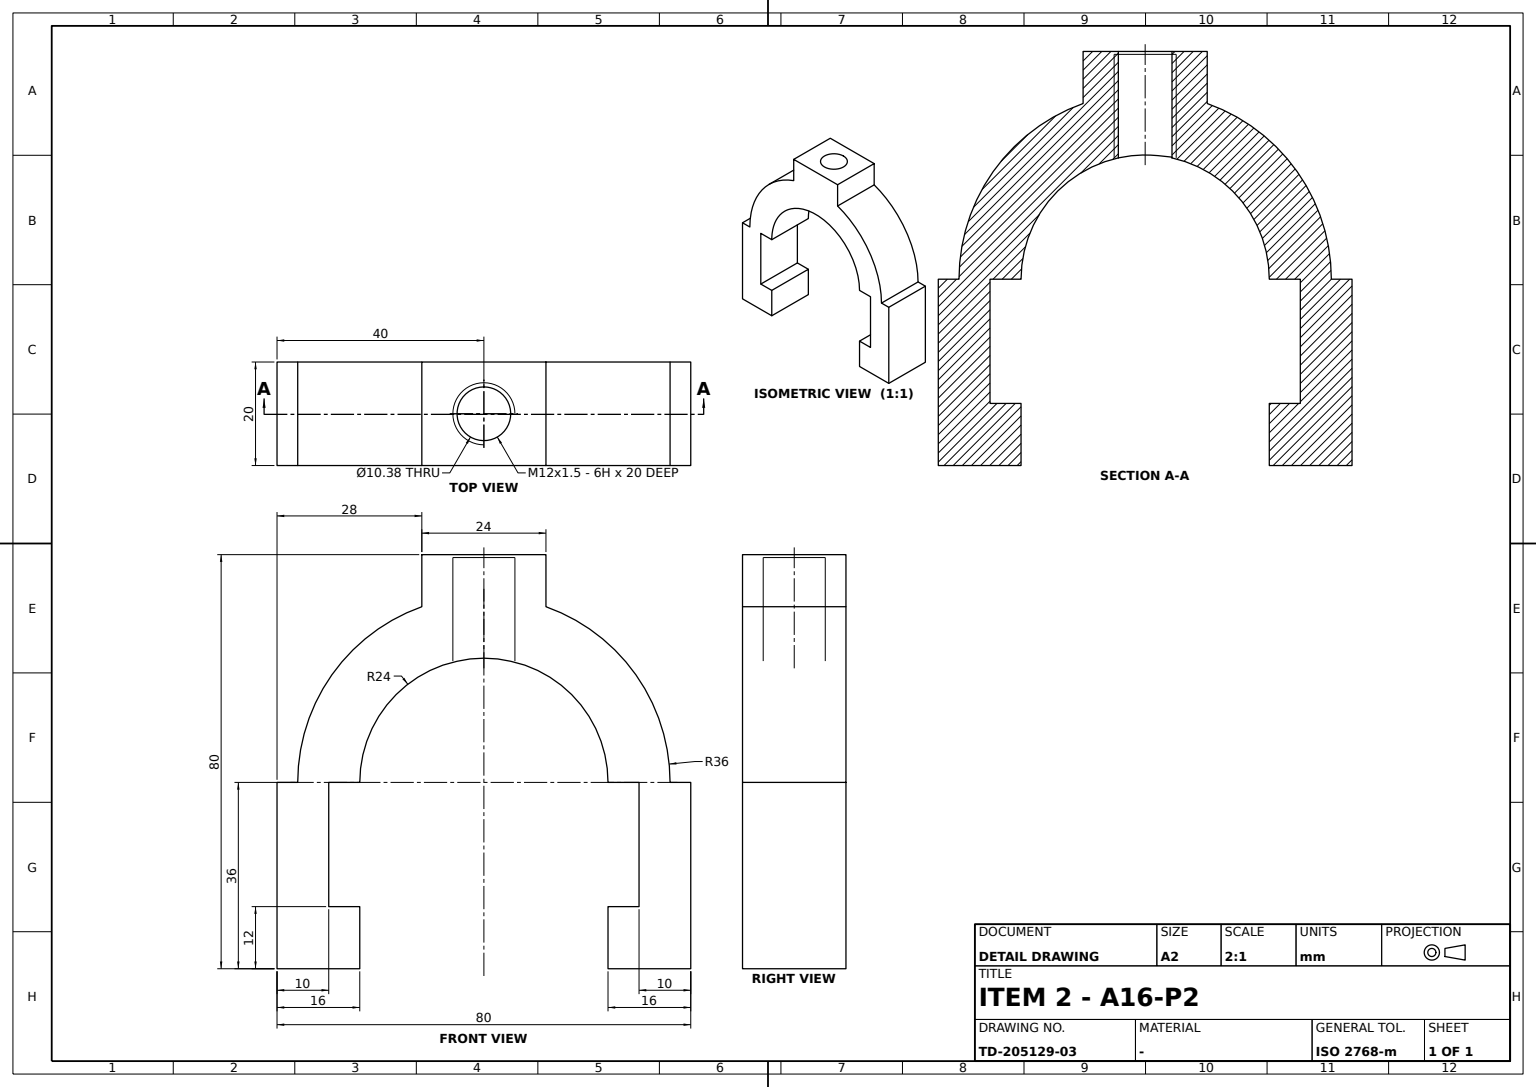
ISO-10303-21;
HEADER;
FILE_DESCRIPTION((''),'2;1');
FILE_NAME('','',(''),(''),'','','');
FILE_SCHEMA(('AUTOMOTIVE_DESIGN'));
ENDSEC;
DATA;
#1=APPLICATION_CONTEXT('');
#2=PRODUCT_CONTEXT('',#1,'mechanical');
#3=PRODUCT('','','',(#2));
#4=PRODUCT_DEFINITION_FORMATION('','',#3);
#5=PRODUCT_DEFINITION_CONTEXT('',#1,'design');
#6=PRODUCT_DEFINITION('','',#4,#5);
#7=PRODUCT_DEFINITION_SHAPE('','',#6);
#8=(LENGTH_UNIT()NAMED_UNIT(*)SI_UNIT(.MILLI.,.METRE.));
#9=(NAMED_UNIT(*)PLANE_ANGLE_UNIT()SI_UNIT($,.RADIAN.));
#10=(NAMED_UNIT(*)SI_UNIT($,.STERADIAN.)SOLID_ANGLE_UNIT());
#11=UNCERTAINTY_MEASURE_WITH_UNIT(LENGTH_MEASURE(0.005),#8,'distance_accuracy_value','');
#12=(GEOMETRIC_REPRESENTATION_CONTEXT(3)GLOBAL_UNCERTAINTY_ASSIGNED_CONTEXT((#11))GLOBAL_UNIT_ASSIGNED_CONTEXT((#8,#9,#10))REPRESENTATION_CONTEXT('',''));
#13=CARTESIAN_POINT('',(0.,24.,0.));
#14=VERTEX_POINT('',#13);
#15=CARTESIAN_POINT('',(0.,40.,0.));
#16=VERTEX_POINT('',#15);
#17=CARTESIAN_POINT('',(0.,0.,0.));
#18=DIRECTION('',(0.,1.,0.));
#19=VECTOR('',#18,1000.);
#20=LINE('',#17,#19);
#21=EDGE_CURVE('',#14,#16,#20,.T.);
#22=ORIENTED_EDGE('',*,*,#21,.T.);
#23=CARTESIAN_POINT('',(20.,40.,0.));
#24=VERTEX_POINT('',#23);
#25=DIRECTION('',(1.,0.,0.));
#26=VECTOR('',#25,1000.);
#27=LINE('',#15,#26);
#28=EDGE_CURVE('',#16,#24,#27,.T.);
#29=ORIENTED_EDGE('',*,*,#28,.T.);
#30=CARTESIAN_POINT('',(20.,24.,0.));
#31=VERTEX_POINT('',#30);
#32=CARTESIAN_POINT('',(20.,0.,0.));
#33=LINE('',#32,#19);
#34=EDGE_CURVE('',#31,#24,#33,.T.);
#35=ORIENTED_EDGE('',*,*,#34,.F.);
#36=LINE('',#13,#26);
#37=EDGE_CURVE('',#14,#31,#36,.T.);
#38=ORIENTED_EDGE('',*,*,#37,.F.);
#39=EDGE_LOOP('',(#22,#29,#35,#38));
#40=FACE_BOUND('',#39,.T.);
#41=DIRECTION('',(0.,0.,-1.));
#42=AXIS2_PLACEMENT_3D('',#13,#41,#18);
#43=PLANE('',#42);
#44=ADVANCED_FACE('',(#40),#43,.T.);
#45=CARTESIAN_POINT('',(0.,30.,12.));
#46=VERTEX_POINT('',#45);
#47=CARTESIAN_POINT('',(0.,24.,12.));
#48=VERTEX_POINT('',#47);
#49=CARTESIAN_POINT('',(0.,0.,12.));
#50=DIRECTION('',(0.,-1.,0.));
#51=VECTOR('',#50,1000.);
#52=LINE('',#49,#51);
#53=EDGE_CURVE('',#46,#48,#52,.T.);
#54=ORIENTED_EDGE('',*,*,#53,.T.);
#55=CARTESIAN_POINT('',(20.,24.,12.));
#56=VERTEX_POINT('',#55);
#57=LINE('',#47,#26);
#58=EDGE_CURVE('',#48,#56,#57,.T.);
#59=ORIENTED_EDGE('',*,*,#58,.T.);
#60=CARTESIAN_POINT('',(20.,30.,12.));
#61=VERTEX_POINT('',#60);
#62=CARTESIAN_POINT('',(20.,0.,12.));
#63=LINE('',#62,#51);
#64=EDGE_CURVE('',#61,#56,#63,.T.);
#65=ORIENTED_EDGE('',*,*,#64,.F.);
#66=LINE('',#45,#26);
#67=EDGE_CURVE('',#46,#61,#66,.T.);
#68=ORIENTED_EDGE('',*,*,#67,.F.);
#69=EDGE_LOOP('',(#54,#59,#65,#68));
#70=FACE_BOUND('',#69,.T.);
#71=DIRECTION('',(0.,0.,1.));
#72=AXIS2_PLACEMENT_3D('',#45,#71,#50);
#73=PLANE('',#72);
#74=ADVANCED_FACE('',(#70),#73,.T.);
#75=CARTESIAN_POINT('',(0.,30.,36.));
#76=VERTEX_POINT('',#75);
#77=CARTESIAN_POINT('',(0.,30.,0.));
#78=VECTOR('',#41,1000.);
#79=LINE('',#77,#78);
#80=EDGE_CURVE('',#76,#46,#79,.T.);
#81=ORIENTED_EDGE('',*,*,#80,.F.);
#82=CARTESIAN_POINT('',(0.,24.,36.));
#83=VERTEX_POINT('',#82);
#84=CARTESIAN_POINT('',(0.,0.,36.));
#85=LINE('',#84,#19);
#86=EDGE_CURVE('',#83,#76,#85,.T.);
#87=ORIENTED_EDGE('',*,*,#86,.F.);
#88=CARTESIAN_POINT('',(0.,-24.,36.));
#89=VERTEX_POINT('',#88);
#90=AXIS2_PLACEMENT_3D('',#84,#25,#41);
#91=CIRCLE('',#90,24.);
#92=EDGE_CURVE('',#83,#89,#91,.T.);
#93=ORIENTED_EDGE('',*,*,#92,.T.);
#94=CARTESIAN_POINT('',(0.,-30.,36.));
#95=VERTEX_POINT('',#94);
#96=LINE('',#82,#51);
#97=EDGE_CURVE('',#89,#95,#96,.T.);
#98=ORIENTED_EDGE('',*,*,#97,.T.);
#99=CARTESIAN_POINT('',(0.,-30.,12.));
#100=VERTEX_POINT('',#99);
#101=CARTESIAN_POINT('',(0.,-30.,0.));
#102=LINE('',#101,#78);
#103=EDGE_CURVE('',#95,#100,#102,.T.);
#104=ORIENTED_EDGE('',*,*,#103,.T.);
#105=CARTESIAN_POINT('',(0.,-24.,12.));
#106=VERTEX_POINT('',#105);
#107=LINE('',#45,#19);
#108=EDGE_CURVE('',#100,#106,#107,.T.);
#109=ORIENTED_EDGE('',*,*,#108,.T.);
#110=CARTESIAN_POINT('',(0.,-24.,0.));
#111=VERTEX_POINT('',#110);
#112=LINE('',#110,#78);
#113=EDGE_CURVE('',#106,#111,#112,.T.);
#114=ORIENTED_EDGE('',*,*,#113,.T.);
#115=CARTESIAN_POINT('',(0.,-40.,0.));
#116=VERTEX_POINT('',#115);
#117=LINE('',#13,#51);
#118=EDGE_CURVE('',#111,#116,#117,.T.);
#119=ORIENTED_EDGE('',*,*,#118,.T.);
#120=CARTESIAN_POINT('',(0.,-40.,36.));
#121=VERTEX_POINT('',#120);
#122=VECTOR('',#71,1000.);
#123=LINE('',#115,#122);
#124=EDGE_CURVE('',#116,#121,#123,.T.);
#125=ORIENTED_EDGE('',*,*,#124,.T.);
#126=CARTESIAN_POINT('',(0.,-36.,36.));
#127=VERTEX_POINT('',#126);
#128=EDGE_CURVE('',#121,#127,#85,.T.);
#129=ORIENTED_EDGE('',*,*,#128,.T.);
#130=CARTESIAN_POINT('',(0.,-12.,69.941125));
#131=VERTEX_POINT('',#130);
#132=CIRCLE('',#90,36.);
#133=EDGE_CURVE('',#131,#127,#132,.T.);
#134=ORIENTED_EDGE('',*,*,#133,.F.);
#135=CARTESIAN_POINT('',(0.,-12.,80.));
#136=VERTEX_POINT('',#135);
#137=CARTESIAN_POINT('',(0.,-12.,0.));
#138=LINE('',#137,#122);
#139=EDGE_CURVE('',#131,#136,#138,.T.);
#140=ORIENTED_EDGE('',*,*,#139,.T.);
#141=CARTESIAN_POINT('',(0.,12.,80.));
#142=VERTEX_POINT('',#141);
#143=CARTESIAN_POINT('',(0.,0.,80.));
#144=LINE('',#143,#19);
#145=EDGE_CURVE('',#136,#142,#144,.T.);
#146=ORIENTED_EDGE('',*,*,#145,.T.);
#147=CARTESIAN_POINT('',(0.,12.,69.941125));
#148=VERTEX_POINT('',#147);
#149=CARTESIAN_POINT('',(0.,12.,0.));
#150=LINE('',#149,#78);
#151=EDGE_CURVE('',#142,#148,#150,.T.);
#152=ORIENTED_EDGE('',*,*,#151,.T.);
#153=CARTESIAN_POINT('',(0.,36.,36.));
#154=VERTEX_POINT('',#153);
#155=EDGE_CURVE('',#154,#148,#132,.T.);
#156=ORIENTED_EDGE('',*,*,#155,.F.);
#157=CARTESIAN_POINT('',(0.,40.,36.));
#158=VERTEX_POINT('',#157);
#159=EDGE_CURVE('',#158,#154,#96,.T.);
#160=ORIENTED_EDGE('',*,*,#159,.F.);
#161=LINE('',#15,#122);
#162=EDGE_CURVE('',#16,#158,#161,.T.);
#163=ORIENTED_EDGE('',*,*,#162,.F.);
#164=ORIENTED_EDGE('',*,*,#21,.F.);
#165=LINE('',#13,#78);
#166=EDGE_CURVE('',#48,#14,#165,.T.);
#167=ORIENTED_EDGE('',*,*,#166,.F.);
#168=ORIENTED_EDGE('',*,*,#53,.F.);
#169=EDGE_LOOP('',(#81,#87,#93,#98,#104,#109,#114,#119,#125,#129,#134,#140,#146,#152,#156,#160,#163,#164,#167,#168));
#170=FACE_BOUND('',#169,.T.);
#171=AXIS2_PLACEMENT_3D('',#17,#25,#18);
#172=PLANE('',#171);
#173=ADVANCED_FACE('',(#170),#172,.F.);
#174=CARTESIAN_POINT('',(20.,-30.,12.));
#175=VERTEX_POINT('',#174);
#176=LINE('',#99,#26);
#177=EDGE_CURVE('',#100,#175,#176,.T.);
#178=ORIENTED_EDGE('',*,*,#177,.F.);
#179=ORIENTED_EDGE('',*,*,#103,.F.);
#180=CARTESIAN_POINT('',(20.,-30.,36.));
#181=VERTEX_POINT('',#180);
#182=LINE('',#94,#26);
#183=EDGE_CURVE('',#95,#181,#182,.T.);
#184=ORIENTED_EDGE('',*,*,#183,.T.);
#185=CARTESIAN_POINT('',(20.,-30.,0.));
#186=LINE('',#185,#78);
#187=EDGE_CURVE('',#181,#175,#186,.T.);
#188=ORIENTED_EDGE('',*,*,#187,.T.);
#189=EDGE_LOOP('',(#178,#179,#184,#188));
#190=FACE_BOUND('',#189,.T.);
#191=AXIS2_PLACEMENT_3D('',#94,#50,#41);
#192=PLANE('',#191);
#193=ADVANCED_FACE('',(#190),#192,.F.);
#194=ORIENTED_EDGE('',*,*,#108,.F.);
#195=ORIENTED_EDGE('',*,*,#177,.T.);
#196=CARTESIAN_POINT('',(20.,-24.,12.));
#197=VERTEX_POINT('',#196);
#198=LINE('',#60,#19);
#199=EDGE_CURVE('',#175,#197,#198,.T.);
#200=ORIENTED_EDGE('',*,*,#199,.T.);
#201=LINE('',#105,#26);
#202=EDGE_CURVE('',#106,#197,#201,.T.);
#203=ORIENTED_EDGE('',*,*,#202,.F.);
#204=EDGE_LOOP('',(#194,#195,#200,#203));
#205=FACE_BOUND('',#204,.T.);
#206=ADVANCED_FACE('',(#205),#73,.T.);
#207=CARTESIAN_POINT('',(20.,30.,36.));
#208=VERTEX_POINT('',#207);
#209=LINE('',#75,#26);
#210=EDGE_CURVE('',#76,#208,#209,.T.);
#211=ORIENTED_EDGE('',*,*,#210,.T.);
#212=CARTESIAN_POINT('',(20.,24.,36.));
#213=VERTEX_POINT('',#212);
#214=CARTESIAN_POINT('',(20.,0.,36.));
#215=LINE('',#214,#19);
#216=EDGE_CURVE('',#213,#208,#215,.T.);
#217=ORIENTED_EDGE('',*,*,#216,.F.);
#218=LINE('',#82,#26);
#219=EDGE_CURVE('',#83,#213,#218,.T.);
#220=ORIENTED_EDGE('',*,*,#219,.F.);
#221=ORIENTED_EDGE('',*,*,#86,.T.);
#222=EDGE_LOOP('',(#211,#217,#220,#221));
#223=FACE_BOUND('',#222,.T.);
#224=AXIS2_PLACEMENT_3D('',#82,#41,#18);
#225=PLANE('',#224);
#226=ADVANCED_FACE('',(#223),#225,.T.);
#227=CARTESIAN_POINT('',(20.,12.,80.));
#228=VERTEX_POINT('',#227);
#229=CARTESIAN_POINT('',(20.,12.,69.941125));
#230=VERTEX_POINT('',#229);
#231=CARTESIAN_POINT('',(20.,12.,0.));
#232=LINE('',#231,#78);
#233=EDGE_CURVE('',#228,#230,#232,.T.);
#234=ORIENTED_EDGE('',*,*,#233,.T.);
#235=LINE('',#147,#26);
#236=EDGE_CURVE('',#148,#230,#235,.T.);
#237=ORIENTED_EDGE('',*,*,#236,.F.);
#238=ORIENTED_EDGE('',*,*,#151,.F.);
#239=LINE('',#141,#26);
#240=EDGE_CURVE('',#142,#228,#239,.T.);
#241=ORIENTED_EDGE('',*,*,#240,.T.);
#242=EDGE_LOOP('',(#234,#237,#238,#241));
#243=FACE_BOUND('',#242,.T.);
#244=AXIS2_PLACEMENT_3D('',#141,#50,#41);
#245=PLANE('',#244);
#246=ADVANCED_FACE('',(#243),#245,.F.);
#247=CARTESIAN_POINT('',(20.,40.,36.));
#248=VERTEX_POINT('',#247);
#249=LINE('',#23,#122);
#250=EDGE_CURVE('',#24,#248,#249,.T.);
#251=ORIENTED_EDGE('',*,*,#250,.F.);
#252=ORIENTED_EDGE('',*,*,#28,.F.);
#253=ORIENTED_EDGE('',*,*,#162,.T.);
#254=LINE('',#157,#26);
#255=EDGE_CURVE('',#158,#248,#254,.T.);
#256=ORIENTED_EDGE('',*,*,#255,.T.);
#257=EDGE_LOOP('',(#251,#252,#253,#256));
#258=FACE_BOUND('',#257,.T.);
#259=AXIS2_PLACEMENT_3D('',#15,#18,#71);
#260=PLANE('',#259);
#261=ADVANCED_FACE('',(#258),#260,.T.);
#262=ORIENTED_EDGE('',*,*,#155,.T.);
#263=ORIENTED_EDGE('',*,*,#236,.T.);
#264=CARTESIAN_POINT('',(20.,36.,36.));
#265=VERTEX_POINT('',#264);
#266=AXIS2_PLACEMENT_3D('',#214,#25,#41);
#267=CIRCLE('',#266,36.);
#268=EDGE_CURVE('',#265,#230,#267,.T.);
#269=ORIENTED_EDGE('',*,*,#268,.F.);
#270=LINE('',#153,#26);
#271=EDGE_CURVE('',#154,#265,#270,.T.);
#272=ORIENTED_EDGE('',*,*,#271,.F.);
#273=EDGE_LOOP('',(#262,#263,#269,#272));
#274=FACE_BOUND('',#273,.T.);
#275=CARTESIAN_POINT('',(10.,0.,36.));
#276=AXIS2_PLACEMENT_3D('',#275,#25,#18);
#277=CYLINDRICAL_SURFACE('',#276,36.);
#278=ADVANCED_FACE('',(#274),#277,.T.);
#279=CARTESIAN_POINT('',(20.,-24.,36.));
#280=VERTEX_POINT('',#279);
#281=LINE('',#212,#51);
#282=EDGE_CURVE('',#280,#181,#281,.T.);
#283=ORIENTED_EDGE('',*,*,#282,.T.);
#284=ORIENTED_EDGE('',*,*,#183,.F.);
#285=ORIENTED_EDGE('',*,*,#97,.F.);
#286=LINE('',#88,#26);
#287=EDGE_CURVE('',#89,#280,#286,.T.);
#288=ORIENTED_EDGE('',*,*,#287,.T.);
#289=EDGE_LOOP('',(#283,#284,#285,#288));
#290=FACE_BOUND('',#289,.T.);
#291=ADVANCED_FACE('',(#290),#225,.T.);
#292=CARTESIAN_POINT('',(20.,-12.,80.));
#293=VERTEX_POINT('',#292);
#294=CARTESIAN_POINT('',(20.,0.,80.));
#295=LINE('',#294,#19);
#296=EDGE_CURVE('',#293,#228,#295,.T.);
#297=ORIENTED_EDGE('',*,*,#296,.T.);
#298=ORIENTED_EDGE('',*,*,#240,.F.);
#299=ORIENTED_EDGE('',*,*,#145,.F.);
#300=LINE('',#135,#26);
#301=EDGE_CURVE('',#136,#293,#300,.T.);
#302=ORIENTED_EDGE('',*,*,#301,.T.);
#303=EDGE_LOOP('',(#297,#298,#299,#302));
#304=FACE_BOUND('',#303,.T.);
#305=CARTESIAN_POINT('',(4.812,0.,80.));
#306=VERTEX_POINT('',#305);
#307=CARTESIAN_POINT('',(10.,0.,80.));
#308=DIRECTION('',(-1.,0.,0.));
#309=AXIS2_PLACEMENT_3D('',#307,#41,#308);
#310=CIRCLE('',#309,5.188);
#311=EDGE_CURVE('',#306,#306,#310,.T.);
#312=ORIENTED_EDGE('',*,*,#311,.T.);
#313=EDGE_LOOP('',(#312));
#314=FACE_BOUND('',#313,.T.);
#315=AXIS2_PLACEMENT_3D('',#135,#41,#18);
#316=PLANE('',#315);
#317=ADVANCED_FACE('',(#304,#314),#316,.F.);
#318=CARTESIAN_POINT('',(20.,-12.,69.941125));
#319=VERTEX_POINT('',#318);
#320=CARTESIAN_POINT('',(20.,-36.,36.));
#321=VERTEX_POINT('',#320);
#322=EDGE_CURVE('',#319,#321,#267,.T.);
#323=ORIENTED_EDGE('',*,*,#322,.F.);
#324=LINE('',#130,#26);
#325=EDGE_CURVE('',#131,#319,#324,.T.);
#326=ORIENTED_EDGE('',*,*,#325,.F.);
#327=ORIENTED_EDGE('',*,*,#133,.T.);
#328=LINE('',#126,#26);
#329=EDGE_CURVE('',#127,#321,#328,.T.);
#330=ORIENTED_EDGE('',*,*,#329,.T.);
#331=EDGE_LOOP('',(#323,#326,#327,#330));
#332=FACE_BOUND('',#331,.T.);
#333=ADVANCED_FACE('',(#332),#277,.T.);
#334=CARTESIAN_POINT('',(5.447102,2.48726,59.870767));
#335=VERTEX_POINT('',#334);
#336=CARTESIAN_POINT('',(4.487008,-1.636267,60.073346));
#337=CARTESIAN_POINT('',(4.95632,2.761937,59.948111));
#338=CARTESIAN_POINT('',(8.37032,5.512077,59.358813));
#339=CARTESIAN_POINT('',(12.754043,5.045498,59.487623));
#340=CARTESIAN_POINT('',(15.512689,1.636626,60.073273));
#341=CARTESIAN_POINT('',(15.044231,-2.760932,59.94824));
#342=CARTESIAN_POINT('',(11.630135,-5.512137,59.358823));
#343=CARTESIAN_POINT('',(7.245919,-5.045572,59.487602));
#344=B_SPLINE_CURVE_WITH_KNOTS('',3,(#336,#337,#338,#339,#340,#341,#342,#343,#336,#337,#338),.UNSPECIFIED.,.T.,.F.,(1,1,1,1,1,1,1,1,1,1,1,1,1,1,1),(-0.012196704,-0.008131136,-0.004065568,0.,0.004065568,0.008131136,0.012196704,0.016262272,0.02032784,0.024393408,0.028458976,0.032524544,0.036590112,0.04065568,0.044721248),.UNSPECIFIED.);
#345=EDGE_CURVE('',#335,#335,#344,.T.);
#346=ORIENTED_EDGE('',*,*,#345,.T.);
#347=EDGE_LOOP('',(#346));
#348=FACE_BOUND('',#347,.T.);
#349=ORIENTED_EDGE('',*,*,#311,.F.);
#350=EDGE_LOOP('',(#349));
#351=FACE_BOUND('',#350,.T.);
#352=CARTESIAN_POINT('',(10.,0.,79.9));
#353=AXIS2_PLACEMENT_3D('',#352,#41,#25);
#354=CYLINDRICAL_SURFACE('',#353,5.188);
#355=ADVANCED_FACE('',(#348,#351),#354,.F.);
#356=ORIENTED_EDGE('',*,*,#124,.F.);
#357=CARTESIAN_POINT('',(20.,-40.,0.));
#358=VERTEX_POINT('',#357);
#359=LINE('',#115,#26);
#360=EDGE_CURVE('',#116,#358,#359,.T.);
#361=ORIENTED_EDGE('',*,*,#360,.T.);
#362=CARTESIAN_POINT('',(20.,-40.,36.));
#363=VERTEX_POINT('',#362);
#364=LINE('',#357,#122);
#365=EDGE_CURVE('',#358,#363,#364,.T.);
#366=ORIENTED_EDGE('',*,*,#365,.T.);
#367=LINE('',#120,#26);
#368=EDGE_CURVE('',#121,#363,#367,.T.);
#369=ORIENTED_EDGE('',*,*,#368,.F.);
#370=EDGE_LOOP('',(#356,#361,#366,#369));
#371=FACE_BOUND('',#370,.T.);
#372=AXIS2_PLACEMENT_3D('',#115,#18,#71);
#373=PLANE('',#372);
#374=ADVANCED_FACE('',(#371),#373,.F.);
#375=CARTESIAN_POINT('',(20.,-24.,0.));
#376=VERTEX_POINT('',#375);
#377=LINE('',#110,#26);
#378=EDGE_CURVE('',#111,#376,#377,.T.);
#379=ORIENTED_EDGE('',*,*,#378,.T.);
#380=LINE('',#30,#51);
#381=EDGE_CURVE('',#376,#358,#380,.T.);
#382=ORIENTED_EDGE('',*,*,#381,.T.);
#383=ORIENTED_EDGE('',*,*,#360,.F.);
#384=ORIENTED_EDGE('',*,*,#118,.F.);
#385=EDGE_LOOP('',(#379,#382,#383,#384));
#386=FACE_BOUND('',#385,.T.);
#387=ADVANCED_FACE('',(#386),#43,.T.);
#388=EDGE_CURVE('',#363,#321,#215,.T.);
#389=ORIENTED_EDGE('',*,*,#388,.T.);
#390=ORIENTED_EDGE('',*,*,#329,.F.);
#391=ORIENTED_EDGE('',*,*,#128,.F.);
#392=ORIENTED_EDGE('',*,*,#368,.T.);
#393=EDGE_LOOP('',(#389,#390,#391,#392));
#394=FACE_BOUND('',#393,.T.);
#395=ADVANCED_FACE('',(#394),#225,.F.);
#396=ORIENTED_EDGE('',*,*,#202,.T.);
#397=LINE('',#375,#78);
#398=EDGE_CURVE('',#197,#376,#397,.T.);
#399=ORIENTED_EDGE('',*,*,#398,.T.);
#400=ORIENTED_EDGE('',*,*,#378,.F.);
#401=ORIENTED_EDGE('',*,*,#113,.F.);
#402=EDGE_LOOP('',(#396,#399,#400,#401));
#403=FACE_BOUND('',#402,.T.);
#404=AXIS2_PLACEMENT_3D('',#105,#50,#41);
#405=PLANE('',#404);
#406=ADVANCED_FACE('',(#403),#405,.F.);
#407=ORIENTED_EDGE('',*,*,#271,.T.);
#408=EDGE_CURVE('',#248,#265,#281,.T.);
#409=ORIENTED_EDGE('',*,*,#408,.F.);
#410=ORIENTED_EDGE('',*,*,#255,.F.);
#411=ORIENTED_EDGE('',*,*,#159,.T.);
#412=EDGE_LOOP('',(#407,#409,#410,#411));
#413=FACE_BOUND('',#412,.T.);
#414=ADVANCED_FACE('',(#413),#225,.F.);
#415=ORIENTED_EDGE('',*,*,#398,.F.);
#416=ORIENTED_EDGE('',*,*,#199,.F.);
#417=ORIENTED_EDGE('',*,*,#187,.F.);
#418=ORIENTED_EDGE('',*,*,#282,.F.);
#419=CIRCLE('',#266,24.);
#420=EDGE_CURVE('',#213,#280,#419,.T.);
#421=ORIENTED_EDGE('',*,*,#420,.F.);
#422=ORIENTED_EDGE('',*,*,#216,.T.);
#423=CARTESIAN_POINT('',(20.,30.,0.));
#424=LINE('',#423,#78);
#425=EDGE_CURVE('',#208,#61,#424,.T.);
#426=ORIENTED_EDGE('',*,*,#425,.T.);
#427=ORIENTED_EDGE('',*,*,#64,.T.);
#428=LINE('',#30,#78);
#429=EDGE_CURVE('',#56,#31,#428,.T.);
#430=ORIENTED_EDGE('',*,*,#429,.T.);
#431=ORIENTED_EDGE('',*,*,#34,.T.);
#432=ORIENTED_EDGE('',*,*,#250,.T.);
#433=ORIENTED_EDGE('',*,*,#408,.T.);
#434=ORIENTED_EDGE('',*,*,#268,.T.);
#435=ORIENTED_EDGE('',*,*,#233,.F.);
#436=ORIENTED_EDGE('',*,*,#296,.F.);
#437=CARTESIAN_POINT('',(20.,-12.,0.));
#438=LINE('',#437,#122);
#439=EDGE_CURVE('',#319,#293,#438,.T.);
#440=ORIENTED_EDGE('',*,*,#439,.F.);
#441=ORIENTED_EDGE('',*,*,#322,.T.);
#442=ORIENTED_EDGE('',*,*,#388,.F.);
#443=ORIENTED_EDGE('',*,*,#365,.F.);
#444=ORIENTED_EDGE('',*,*,#381,.F.);
#445=EDGE_LOOP('',(#415,#416,#417,#418,#421,#422,#426,#427,#430,#431,#432,#433,#434,#435,#436,#440,#441,#442,#443,#444));
#446=FACE_BOUND('',#445,.T.);
#447=AXIS2_PLACEMENT_3D('',#32,#25,#18);
#448=PLANE('',#447);
#449=ADVANCED_FACE('',(#446),#448,.T.);
#450=ORIENTED_EDGE('',*,*,#325,.T.);
#451=ORIENTED_EDGE('',*,*,#439,.T.);
#452=ORIENTED_EDGE('',*,*,#301,.F.);
#453=ORIENTED_EDGE('',*,*,#139,.F.);
#454=EDGE_LOOP('',(#450,#451,#452,#453));
#455=FACE_BOUND('',#454,.T.);
#456=AXIS2_PLACEMENT_3D('',#130,#18,#71);
#457=PLANE('',#456);
#458=ADVANCED_FACE('',(#455),#457,.F.);
#459=ORIENTED_EDGE('',*,*,#429,.F.);
#460=ORIENTED_EDGE('',*,*,#58,.F.);
#461=ORIENTED_EDGE('',*,*,#166,.T.);
#462=ORIENTED_EDGE('',*,*,#37,.T.);
#463=EDGE_LOOP('',(#459,#460,#461,#462));
#464=FACE_BOUND('',#463,.T.);
#465=AXIS2_PLACEMENT_3D('',#47,#50,#41);
#466=PLANE('',#465);
#467=ADVANCED_FACE('',(#464),#466,.T.);
#468=ORIENTED_EDGE('',*,*,#420,.T.);
#469=ORIENTED_EDGE('',*,*,#287,.F.);
#470=ORIENTED_EDGE('',*,*,#92,.F.);
#471=ORIENTED_EDGE('',*,*,#219,.T.);
#472=EDGE_LOOP('',(#468,#469,#470,#471));
#473=FACE_BOUND('',#472,.T.);
#474=ORIENTED_EDGE('',*,*,#345,.F.);
#475=EDGE_LOOP('',(#474));
#476=FACE_BOUND('',#475,.T.);
#477=CYLINDRICAL_SURFACE('',#276,24.);
#478=ADVANCED_FACE('',(#473,#476),#477,.F.);
#479=ORIENTED_EDGE('',*,*,#425,.F.);
#480=ORIENTED_EDGE('',*,*,#210,.F.);
#481=ORIENTED_EDGE('',*,*,#80,.T.);
#482=ORIENTED_EDGE('',*,*,#67,.T.);
#483=EDGE_LOOP('',(#479,#480,#481,#482));
#484=FACE_BOUND('',#483,.T.);
#485=AXIS2_PLACEMENT_3D('',#75,#50,#41);
#486=PLANE('',#485);
#487=ADVANCED_FACE('',(#484),#486,.T.);
#488=CLOSED_SHELL('',(#44,#74,#173,#193,#206,#226,#246,#261,#278,#291,#317,#333,#355,#374,#387,#395,#406,#414,#449,#458,#467,#478,#487));
#489=MANIFOLD_SOLID_BREP('',#488);
#490=ADVANCED_BREP_SHAPE_REPRESENTATION('',(#489),#12);
#491=SHAPE_DEFINITION_REPRESENTATION(#7,#490);
ENDSEC;
END-ISO-10303-21;
